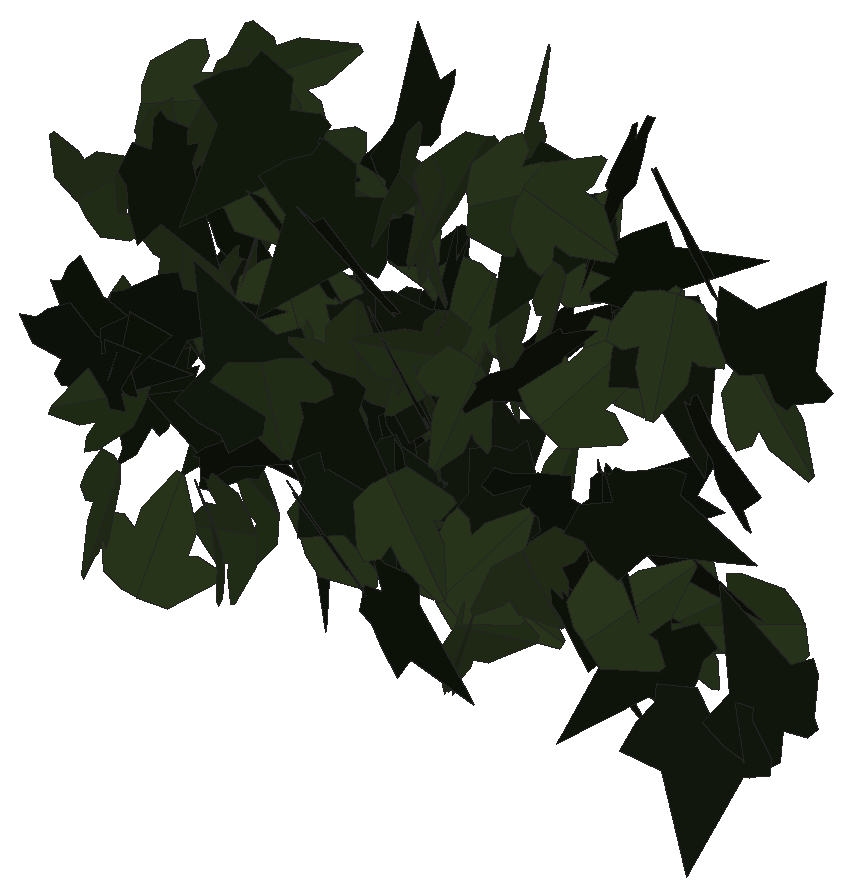
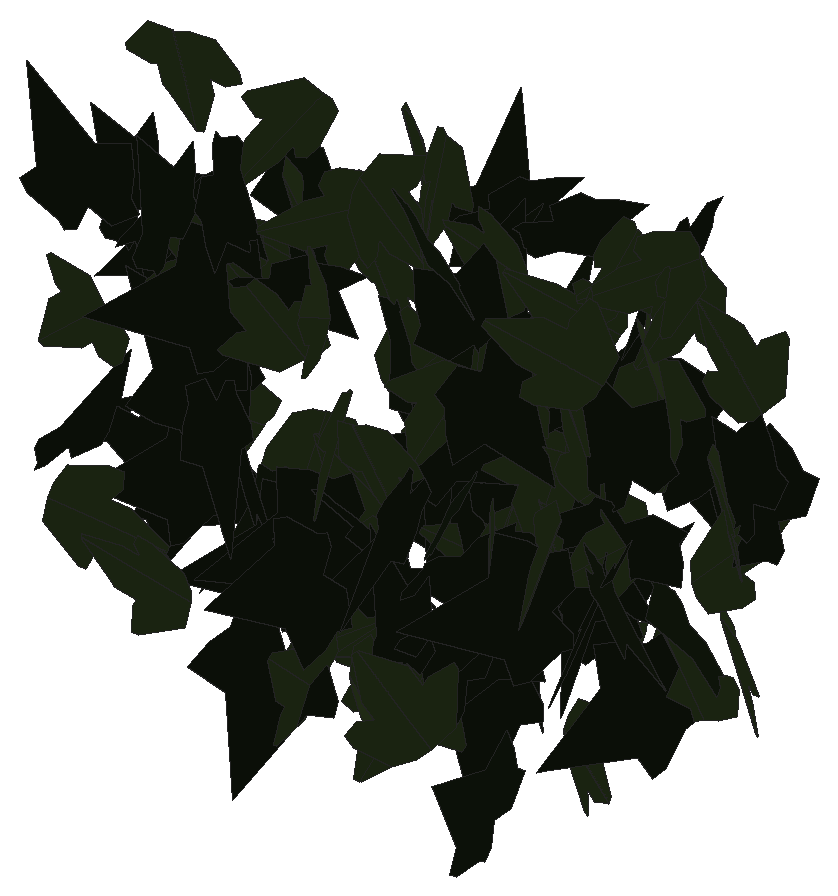
# SketchUp Ruby script. Lengths in inches.
U = 1.inch
M = Sketchup.active_model
def pt(a) = Geom::Point3d.new(a.map { |v| v * U })
def face(e, loops, mat)
  f = e.add_face(loops[0].map { |a| pt(a) })
  loops[1..].each { |l| e.add_face(l.map { |a| pt(a) }).erase! }
  f.material = f.back_material = mat if mat
  f
end
# faces: each face lists its corners as indices into pts; further lists are holes
def faces(e, pts, list, mat = nil) = list.each { |f| face(e, (f[0].is_a?(Array) ? f : [f]).map { |l| l.map { |i| pts[i] } }, mat) }
# xy, xz, yz: faces in a plane at the given z, y or x. An outline is a flat list of corners, or four numbers for a rectangle; further outlines are holes
def ring(l) = l.size == 4 ? [[l[0], l[1]], [l[2], l[1]], [l[2], l[3]], [l[0], l[3]]] : l.each_slice(2).to_a
def flat(e, list, mat, &to3) = list.each { |f| face(e, (f[0].is_a?(Array) ? f : [f]).map { |l| ring(l).map { |u, v| to3.(u, v) } }, mat) }
def xy(e, z, list, mat = nil) = flat(e, list, mat) { |x, y| [x, y, z] }
def xz(e, y, list, mat = nil) = flat(e, list, mat) { |x, z| [x, y, z] }
def yz(e, x, list, mat = nil) = flat(e, list, mat) { |y, z| [x, y, z] }
def lines(e, pts, list) = list.each { |a, b| e.add_line(pt(pts[a]), pt(pts[b])) }
# prism: a flat outline (further loops are holes) pulled along v
def prism(e, loops, v, mat = nil)
  f = face(e, loops, mat); d = Geom::Vector3d.new(v.map { |x| x * U })
  f.pushpull(f.normal.samedirection?(d) ? d.length : -d.length)
end
def box(e, o, s, mat = nil) = prism(e, [[o, [o[0] + s[0], o[1], o[2]], [o[0] + s[0], o[1] + s[1], o[2]], [o[0], o[1] + s[1], o[2]]]], [0, 0, s[2]], mat)
def at(x, y, z, deg = 0) = Geom::Transformation.translation(pt([x, y, z])) * Geom::Transformation.rotation(ORIGIN, Z_AXIS, deg.degrees)
def axes(o, x, y, z) = Geom::Transformation.new([*x, 0, *y, 0, *z, 0, *pt(o).to_a, 1])
def part(name) = M.definitions.add(name)
# library, detail: a bought-in or finely detailed component or shape, given as its bounding box
def library(name, o, s) = part(name).tap { |d| box(d.entities, o, s) }
def detail(e, o, s) = box(e.add_group.entities, o, s)
def put(e, d, t, mat = nil) = e.add_instance(d, t).tap { |i| i.material = mat if mat }
def group(e, t, mat = nil) = e.add_group.tap { |g| g.transformation = t; g.material = mat if mat }.entities
root = M.entities
M.materials.add("efeu1").color = [18, 25, 13]
M.materials.add("efeu2").color = [43, 57, 29]
c1 = part("ivyleaf_9")
p = [[1.54,2.16,1.25],[1.36,2.04,1.19],[-0.21,0.99,0.68],[-0.71,1.11,0.82],[-0.85,0.86,0.67],[-0.8,0.17,0.21],
  [-0.9,-0.01,0.1],[-0.67,-0.16,-0.02],[-0.08,-0.08,-0.05],[-0.03,-0.6,-0.4],[0.65,-0.88,-0.66],[0.83,-0.6,-0.49],
  [1.29,-0.42,-0.43],[1.8125,-0.07,-0.26],[1.21,0.44,0.15]]
faces(c1.entities,p,[[0,1,2,3,4,5,6,7,8,9,10,11,12,13,14]],"efeu1")
c2 = part("ivyleaf_10")
p = [[0,0.5,-0.03],[-0.0625,2.02,-0.43],[-0.19,2.01,-0.46],[-0.54,1.05,-0.29],[-0.52,0.625,-0.18],[-0.83,0.76,-0.28],
  [-1.16,0.64,-0.33],[-1.15,0.33,-0.24],[-0.77,-0.39,0.02],[-0.3,-0.51,0.16],[0.04,-0.48,0.23],[-0.02,2.01,-0.4375],
  [-0.06,2.01,-0.43],[0.04,-0.49,0.23],[0.67,-0.49,0.14],[1.38,0.36,-0.2],[1.375,0.51,-0.24],[0.81,0.65,-0.19],
  [0.62,0.59,-0.15],[0.6,1.09,-0.28],[0.5,1.23,-0.31]]
faces(c2.entities,p,[[0,1,2,3,4,5,6,7,8,9,10],[11,12,0,13,14,15,16,17,18,19,20]],"efeu2")
put(root,c1,axes([34.07,223.39,206.13],[0.4384,-0.24034,-0.00644],[0.00838,0.00189,0.49993],[-0.24028,-0.43844,0.00568]))
put(root,c1,axes([31.94,223.07,206.74],[0.22056,-0.30024,-0.33348],[-0.20029,0.26664,-0.37254],[0.40154,0.29792,-0.00265]))
put(root,c1,axes([30.77,223.2,204.06],[0.1906,-0.09686,0.45198],[0.42903,-0.14491,-0.21197],[0.17206,0.46863,0.02787]))
put(root,c1,axes([34.6,223.26,202.79],[0.0717,-0.0025,-0.49483],[0.47484,0.14103,0.06809],[0.13923,-0.47969,0.02259]))
put(root,c2,axes([33.21,223.19,204.7],[-0.40616,-0.28493,-0.06203],[0.05046,0.03608,-0.49614],[0.2872,-0.40929,-0.00056]))
put(root,c1,axes([30.91,223.38,204.3],[0.05748,-0.04069,0.49501],[0.3527,-0.34752,-0.06953],[0.34971,0.35718,-0.01125]))
put(root,c1,axes([33.08,223.3,204.41],[-0.29967,-0.38714,0.10159],[0.07084,0.07361,0.48945],[-0.39393,0.30774,0.01073]))
put(root,c1,axes([37.58,223.06,204.92],[0.02345,0.04725,-0.49721],[0.20159,0.45452,0.0527],[0.45696,-0.20293,0.00226]))
put(root,c2,axes([35.47,223.38,205.33],[0.45672,-0.16892,-0.11347],[-0.1029,0.04882,-0.48686],[0.17556,0.46806,0.00983]))
put(root,c2,axes([31.09,223.42,202.68],[0.36787,-0.33824,-0.01633],[-0.01131,0.01182,-0.49973],[0.33844,0.36804,0.00105]))
put(root,c2,axes([31.08,223.71,203.58],[-0.01321,0.12806,0.48314],[0.05546,-0.47995,0.12873],[0.49674,0.05699,-0.00152]))
put(root,c1,axes([38.33,223.51,202.61],[-0.33617,-0.30777,-0.2056],[0.15204,0.13841,-0.45577],[0.33746,-0.36895,0.00053]))
put(root,c1,axes([33.8125,223.7,206.63],[-0.29437,-0.37516,0.15034],[-0.09391,-0.11741,-0.47686],[0.3931,-0.30898,-0.00134]))
put(root,c2,axes([34.64,223.34,203.78],[0.38218,0.0878,0.3102],[0.2955,0.09696,-0.39151],[-0.12891,0.48259,0.02222]))
put(root,c2,axes([37.89,223.44,206.87],[0.49581,0.06396,-0.00897],[-0.00898,-0.00046,-0.49992],[-0.06396,0.49589,0.0007]))
put(root,c1,axes([33.59,223.33,203.33],[0.45984,-0.15266,-0.12345],[-0.11699,0.03941,-0.48452],[0.15766,0.47449,0.00053]))
put(root,c1,axes([31.59,223.2,204.81],[0.11228,0.265,-0.40886],[0.15349,0.37898,0.28778],[0.46242,-0.19013,0.00375]))
put(root,c1,axes([36.2,223.23,205.86],[0.11141,0.48401,0.05764],[0.01045,0.05674,-0.49666],[-0.48732,0.11188,0.00253]))
put(root,c2,axes([31.14,223.57,204.49],[0.30433,-0.39325,-0.05231],[-0.02972,0.04314,-0.49725],[0.3956,0.30577,0.00288]))
put(root,c2,axes([30.74,223.57,205.66],[-0.35078,-0.05237,0.35244],[0.34824,0.05427,0.35466],[-0.0754,0.49428,-0.00159]))
put(root,c2,axes([32.18,223.72,202.19],[-0.3085,0.23753,0.3137],[0.25062,-0.18868,0.38934],[0.30334,0.39746,-0.00264]))
put(root,c1,axes([38.12,223.85,205.24],[0.08623,-0.14365,0.47109],[0.23735,-0.40694,-0.16753],[0.43155,0.25252,-0.00199]))
put(root,c2,axes([31.5,223.5,201.88],[0.45195,0.15396,-0.14845],[0.13309,0.06923,0.47696],[0.16742,-0.47064,0.02159]))
put(root,c2,axes([34.88,223.61,207.05],[0.30292,-0.3586,-0.17218],[-0.10876,0.13351,-0.46941],[0.38263,0.32184,0.00289]))
put(root,c2,axes([31.86,223.68,205.34],[-0.47292,0.00245,0.1623],[-0.16231,-0.00107,-0.47292],[-0.00197,-0.49999,0.00181]))
put(root,c1,axes([33.3125,223.76,204.23],[0.0215,-0.10125,-0.48917],[0.44127,0.23334,-0.0289],[0.23413,-0.43047,0.09938]))
put(root,c1,axes([32.73,224.0625,207.03],[-0.3723,-0.31172,0.11928],[-0.09291,-0.07484,-0.48556],[0.32057,-0.38371,-0.00219]))
put(root,c2,axes([31.5,223.47,206.47],[-0.09083,-0.25316,-0.4215],[0.11357,0.40624,-0.26846],[0.47839,-0.1445,-0.01629]))
put(root,c2,axes([32.52,223.62,202.6],[0.17773,-0.10158,-0.45617],[-0.3627,0.27779,-0.20317],[0.29472,0.40313,0.02506]))
put(root,c1,axes([36.63,224.04,204.18],[0.06684,-0.04272,-0.49367],[0.49048,-0.06511,0.07204],[-0.07045,-0.4939,0.03321]))
put(root,c2,axes([31.4375,224.16,205.71],[0.00836,-0.11522,-0.48647],[0.24776,-0.42163,0.10412],[-0.43422,-0.2428,0.05004]))
put(root,c2,axes([35.12,223.84,202.42],[0.22829,-0.4181,-0.1519],[-0.05943,0.14054,-0.47615],[0.44085,0.23546,0.01447]))
put(root,c1,axes([33.84,223.89,203.62],[-0.14546,-0.31251,-0.36219],[0.18397,0.3129,-0.34387],[0.44158,-0.2333,0.02396]))
put(root,c2,axes([33.68,223.95,204.54],[-0.49079,-0.07993,0.05232],[0.05206,0.00584,0.49725],[-0.0801,0.49354,0.00259]))
put(root,c2,axes([35.92,223.78,203.39],[-0.21641,-0.40029,-0.2072],[0.10442,0.17907,-0.45501],[0.43848,-0.24021,0.00609]))
put(root,c2,axes([35.08,223.82,202.9],[0.39783,-0.05889,-0.29709],[0.30247,0.05209,0.39471],[-0.01554,-0.49378,0.07707]))
put(root,c2,axes([36.97,223.63,203.15],[0.24053,0.10153,-0.42642],[0.31555,0.29752,0.24882],[0.30426,-0.38881,0.07905]))
put(root,c2,axes([33.43,223.79,202.79],[-0.15112,-0.09875,0.46627],[0.37788,0.27328,0.18035],[-0.29047,0.4069,-0.00797]))
put(root,c2,axes([34.38,224.31,204.86],[-0.16062,-0.14724,-0.45002],[-0.25648,-0.3724,0.21339],[-0.39802,0.2994,0.0441]))
put(root,c2,axes([35.98,224.08,206.17],[0.33213,-0.37264,0.02882],[0.01921,-0.02148,-0.49917],[0.37326,0.33269,0.00005]))
put(root,c2,axes([34.26,224.2,206.37],[0.11398,-0.16037,0.45966],[0.43291,-0.18257,-0.17104],[0.2227,0.43698,0.09724]))
put(root,c1,axes([37.16,224.32,202.8],[-0.04519,0.04954,-0.49548],[0.10819,-0.48466,-0.05832],[-0.48606,-0.11248,0.03308]))
put(root,c2,axes([34.39,224.1875,204.21],[-0.26461,0.1229,0.40605],[0.35228,-0.203,0.29102],[0.23639,0.4401,0.02084]))
put(root,c2,axes([36.3,223.77,205.24],[0.30242,0.13345,-0.37514],[0.29554,0.24045,0.32379],[0.26683,-0.41758,0.06656]))
put(root,c2,axes([34.34,223.8,207.04],[0.03312,-0.33798,-0.36697],[-0.039,0.3649,-0.3396],[0.49737,0.05112,-0.00219]))
put(root,c1,axes([34.13,223.88,205.06],[0.39342,-0.07811,-0.29853],[-0.28881,0.07717,-0.40079],[0.10868,0.4878,0.0156]))
put(root,c1,axes([32.45,223.71,203.56],[0.25626,0.39871,0.15927],[0.08787,0.13285,-0.47395],[-0.42025,0.27089,-0.00198]))
put(root,c1,axes([38.73,224.08,202.48],[-0.21119,-0.41637,0.17899],[0.07731,0.16148,0.46685],[-0.44657,0.22486,-0.00383]))
put(root,c1,axes([32.7,224.39,205.41],[0.35135,-0.35568,0.00652],[-0.00459,0.00464,0.49996],[-0.35571,-0.35138,-0.00001]))
put(root,c2,axes([31.46,223.83,206.85],[-0.02544,-0.08901,-0.49136],[0.34034,0.35693,-0.08228],[0.36541,-0.33864,0.04243]))
put(root,c2,axes([35.15,223.84,202.41],[-0.09021,-0.25578,-0.42005],[0.15535,0.39037,-0.27107],[0.46661,-0.17942,0.00904]))
put(root,c1,axes([33.62,224.3,203.6],[-0.14995,-0.0359,-0.47563],[0.47558,0.02703,-0.15197],[0.03662,-0.49798,0.02604]))
put(root,c1,axes([36.16,224.09,202.86],[0.41553,-0.24357,-0.13418],[-0.11019,0.07731,-0.48154],[0.25533,0.42976,0.01057]))
put(root,c2,axes([33.18,224.29,206.43],[0.00177,0.00283,-0.49999],[0.44477,-0.22842,0.00028],[-0.22842,-0.44476,-0.00333]))
put(root,c2,axes([32.27,224.06,206.05],[0.25037,-0.02872,-0.43185],[0.42726,0.09595,0.24133],[0.06901,-0.48987,0.07259]))
put(root,c2,axes([31.94,223.97,206.92],[-0.03508,-0.28814,-0.40712],[0.0865,0.39843,-0.28944],[0.49121,-0.09074,0.02189]))
put(root,c1,axes([31.99,224.59,203.04],[0.01665,0.00497,0.4997],[-0.392,-0.30996,0.01614],[0.30994,-0.3923,-0.00642]))
put(root,c1,axes([33.5625,224.66,203.77],[0.04799,-0.34459,0.35911],[0.03588,-0.35744,-0.34778],[0.4964,0.05915,-0.00958]))
put(root,c2,axes([35.88,224.0625,207.15],[0.08648,0.33064,0.36497],[0.08023,0.35614,-0.34165],[-0.48589,0.11765,0.00854]))
put(root,c1,axes([33.42,224.49,205.6875],[0.39266,-0.06735,0.30213],[-0.29523,0.06521,0.39823],[-0.09305,-0.49113,0.01144]))
put(root,c1,axes([31.14,224.0625,203.125],[-0.3581,0.30239,-0.17414],[-0.1335,0.11182,0.46869],[0.3224,0.38217,0.00065]))
put(root,c2,axes([34.52,224.65,206.93],[0.01234,-0.43248,0.25062],[0.0019,-0.25065,-0.43263],[0.49984,0.01163,-0.00454]))
put(root,c1,axes([36.65,224.41,203.99],[0.38756,0.31035,-0.05901],[0.04133,0.04279,0.49645],[0.31319,-0.38969,0.00751]))
put(root,c1,axes([37,224.56,205.99],[0.04974,-0.46674,-0.17226],[-0.01821,0.1713,-0.46939],[0.49719,0.05297,0.00004]))
put(root,c1,axes([33.9375,224.76,204.55],[-0.09456,-0.11124,-0.47821],[-0.28459,-0.38442,0.14569],[-0.40008,0.29974,0.00939]))
put(root,c1,axes([32.01,224.84,203.81],[-0.41113,-0.28083,0.0459],[-0.03495,-0.03021,-0.49786],[0.2824,-0.41258,0.0052]))
put(root,c1,axes([32.62,224.73,202.73],[-0.19506,0.02643,-0.45962],[0.45732,-0.04633,-0.19675],[-0.05299,-0.49715,-0.0061]))
put(root,c1,axes([32.42,224.91,202.76],[0.11449,-0.34193,0.34638],[0.15474,-0.3118,-0.35894],[0.46146,0.18939,0.03442]))
put(root,c2,axes([36.6,224.43,205.35],[0.3567,0.23554,-0.25939],[0.21808,0.14046,0.42745],[0.27423,-0.41808,-0.00253]))
put(root,c1,axes([35.02,224.7,203.29],[-0.47854,0.12026,0.08084],[-0.07874,0.01838,-0.49342],[-0.12165,-0.48497,0.00135]))
put(root,c1,axes([31.28,224.78,205.07],[-0.10126,-0.05501,0.48654],[0.3841,-0.31706,0.04409],[0.30367,0.38268,0.10647]))
put(root,c2,axes([32.28,224.73,204.15],[0.43906,-0.23754,-0.02831],[-0.02478,0.01369,-0.4992],[0.23794,0.43976,0.00025]))
put(root,c2,axes([32.69,224.91,205.64],[-0.09555,-0.02774,-0.49],[-0.422,-0.25023,0.09646],[-0.25058,0.43199,0.0244]))
put(root,c1,axes([36.33,224.52,203.48],[-0.09554,0.02319,-0.49024],[-0.48756,0.05265,0.09751],[0.05615,0.49668,0.01255]))
put(root,c2,axes([31.88,224.69,204.95],[0.20578,-0.44901,0.07776],[-0.03267,0.07056,0.49392],[-0.45452,-0.20835,-0.0003]))
put(root,c2,axes([32.23,224.6875,204.74],[0.35938,0.31794,0.14056],[0.10071,0.09828,-0.47979],[-0.33272,0.37317,0.0066]))
put(root,c1,axes([37.97,224.82,205.76],[-0.22435,0.00566,0.44681],[0.37476,-0.2699,0.19159],[0.24335,0.42086,0.11686]))
put(root,c1,axes([35.33,224.6,202.63],[0.38188,0.03497,0.32085],[0.3205,0.0175,-0.38337],[-0.03804,0.49847,-0.00905]))
put(root,c2,axes([33.02,224.62,203.78],[-0.16222,0.45108,0.14216],[-0.054,0.13164,-0.47933],[-0.46986,-0.17087,0.00601]))
put(root,c1,axes([34.27,224.43,205.09],[-0.00781,0.19555,0.46011],[-0.04538,0.45799,-0.19542],[-0.49787,-0.04481,0.01059]))
put(root,c1,axes([31.375,224.77,204.43],[-0.13857,-0.2522,-0.40889],[0.18723,0.36356,-0.2877],[0.44243,-0.23284,-0.00632]))
put(root,c2,axes([34.84,224.5625,206.64],[0.00912,-0.02692,-0.49919],[0.32058,0.38342,-0.01482],[0.38359,-0.31979,0.02425]))
put(root,c2,axes([34.49,224.74,202.27],[0.19487,0.15919,0.43207],[0.34859,0.25553,-0.25137],[-0.30085,0.3992,-0.01139]))
put(root,c1,axes([36.37,224.95,203.34],[0.40085,-0.15359,0.25638],[0.23896,-0.09288,-0.42927],[0.17949,0.46667,-0.00106]))
put(root,c2,axes([31.42,224.62,204.18],[0.05875,-0.0265,0.49583],[-0.07987,0.49228,0.03577],[-0.49007,-0.08341,0.05361]))
put(root,c2,axes([31.96,225.04,206.25],[0.39486,-0.26454,-0.15527],[-0.1191,0.10101,-0.47499],[0.28267,0.41209,0.01675]))
put(root,c1,axes([31.68,224.93,203.9375],[0.34999,-0.03686,-0.35518],[-0.35428,0.02637,-0.35184],[0.04467,0.49794,-0.00766]))
put(root,c1,axes([33.75,224.8,206.78],[-0.37999,0.1841,-0.2678],[-0.24654,0.10512,0.4221],[0.21172,0.45283,0.01089]))
put(root,c1,axes([34.79,224.88,203.17],[0.40532,0.08675,0.27962],[0.27313,0.05992,-0.4145],[-0.10543,0.48876,0.00118]))
put(root,c1,axes([30.77,224.95,202.83],[0.48374,0.03106,0.1226],[0.12239,0.00722,-0.48474],[-0.03188,0.49898,-0.00062]))
put(root,c2,axes([33.51,225.03,202.33],[0.06392,0.02979,0.495],[0.43453,0.23712,-0.07038],[-0.23895,0.43919,0.00442]))
put(root,c1,axes([31.29,225.06,204.03],[0.28125,-0.2618,-0.31993],[-0.23626,0.21574,-0.38424],[0.33923,0.36731,-0.00235]))
put(root,c1,axes([32.63,225.34,205.91],[-0.12453,0.30599,-0.37532],[0.14118,-0.34775,-0.33036],[-0.46321,-0.18826,0.00022]))
put(root,c2,axes([31.73,225.01,202.03],[0.06425,-0.02227,-0.49535],[-0.34018,0.36143,-0.06037],[0.36076,0.34478,0.03129]))
put(root,c2,axes([37.72,225.3,202.68],[0.14309,0.00658,-0.47904],[-0.47907,0.00659,-0.143],[0.00443,0.49991,0.00819]))
put(root,c1,axes([35.03,225.58,206.24],[-0.37434,-0.32981,0.03305],[-0.02345,-0.02338,-0.4989],[0.33063,-0.37507,0.00204]))
put(root,c2,axes([34.62,225.09,204.66],[-0.23098,0.38258,0.22423],[-0.12977,0.18344,-0.44666],[-0.42404,-0.26454,0.01455]))
put(root,c1,axes([36.3,225.625,206.35],[0.07425,-0.19821,0.45299],[0.20342,-0.40526,-0.21067],[0.45067,0.21558,0.02046]))
put(root,c1,axes([35.77,225.55,207.09],[-0.21281,0.17516,-0.41717],[0.32708,-0.25899,-0.27558],[-0.31263,-0.39019,-0.00435]))
put(root,c1,axes([32.66,225.24,202.57],[0.3581,0.19668,-0.28824],[-0.25624,-0.13213,-0.40851],[-0.23686,0.44029,0.00617]))
put(root,c1,axes([31.09,225.5,204.25],[-0.39926,0.17521,-0.24474],[0.21868,-0.11049,-0.43586],[-0.20681,-0.45508,0.0116]))
put(root,c2,axes([32.99,225.26,205.64],[0.22276,0.38519,0.22806],[0.10564,0.2023,-0.44487],[-0.43499,0.24638,0.00874]))
put(root,c2,axes([36.47,225.45,202.24],[0.11999,-0.06868,-0.4805],[0.47682,-0.0759,0.12992],[-0.09079,-0.48941,0.04728]))
put(root,c2,axes([37.32,225.48,205.05],[0.31093,0.03131,0.39031],[0.38718,0.04981,-0.31243],[-0.05845,0.49653,0.00673]))
put(root,c1,axes([34.09,225.45,202.95],[-0.36015,-0.29964,0.17467],[0.13388,0.11219,0.4685],[-0.31995,0.38423,-0.00058]))
put(root,c2,axes([31.45,225.35,206.39],[-0.17827,-0.16865,0.43563],[0.32435,0.29087,0.24534],[-0.33618,0.37007,0.00569]))
put(root,c2,axes([33.88,225.56,204.8],[0.46062,-0.10886,-0.16118],[-0.1553,0.04362,-0.47327],[0.1171,0.48605,0.00637]))
put(root,c1,axes([32.57,225.74,204.11],[-0.08886,-0.48699,-0.07031],[0.01968,0.06788,-0.49498],[0.49165,-0.09074,0.00711]))
put(root,c2,axes([34.93,225.47,205.54],[0.39722,0.09566,-0.28821],[0.28099,0.06415,0.40857],[0.11514,-0.48655,-0.0028]))
put(root,c1,axes([35.68,225.42,205.71],[0.27782,0.11073,0.40069],[0.3581,0.18103,-0.29832],[-0.21114,0.45273,0.02128]))
put(root,c1,axes([32.36,225.98,202.96],[0.15904,-0.22227,0.41869],[0.25358,-0.33324,-0.27322],[0.40051,0.29925,0.00673]))
put(root,c1,axes([32.98,226.13,203.05],[-0.03893,-0.05137,0.49583],[0.24257,-0.43643,-0.02616],[0.43548,0.23851,0.0589]))
put(root,c2,axes([32.26,225.64,204.39],[0.08581,-0.21931,-0.44106],[-0.16091,0.41067,-0.2355],[0.46556,0.18236,-0.0001]))
put(root,c1,axes([32.25,226.01,203.43],[-0.17672,-0.33925,-0.32199],[0.16732,0.27557,-0.38218],[0.43678,-0.24283,0.01613]))
put(root,c1,axes([33.18,225.84,204.5625],[0.15182,-0.05383,-0.47334],[-0.33164,0.34471,-0.14557],[0.342,0.35816,0.06896]))
put(root,c1,axes([34.61,225.98,202.4],[0.30454,0.39263,-0.05566],[-0.04085,-0.03874,-0.49682],[-0.39445,0.30715,0.00848]))
put(root,c2,axes([32.89,226.13,202.65],[-0.38308,-0.22994,-0.22444],[0.19868,0.10498,-0.44666],[0.25253,-0.4314,0.01094]))
put(root,c2,axes([31.37,225.93,204.78],[-0.11958,0.1535,0.46058],[-0.26927,0.37373,-0.19447],[-0.40397,-0.29456,-0.00671]))
put(root,c2,axes([34.08,226.08,206.36],[0.1616,-0.21161,0.42321],[-0.27553,0.32149,0.26595],[-0.38467,-0.31917,-0.0127]))
put(root,c2,axes([34.25,226,202.24],[0.02187,0.31057,-0.39124],[0.04917,0.38838,0.31104],[0.4971,-0.05208,-0.01355]))
put(root,c1,axes([35.22,226.23,205.04],[0.24784,0.03647,-0.43272],[-0.42945,-0.05333,-0.25046],[-0.06442,0.49581,0.00489]))
put(root,c1,axes([31.1,226.3,204.27],[0.37776,0.03737,0.32543],[0.32026,0.06216,-0.3789],[-0.06878,0.49471,0.02303]))
put(root,c2,axes([32.84,226.97,203.09],[0.26632,-0.32374,0.27252],[0.1694,-0.21351,-0.41919],[0.38778,0.31561,-0.00404]))
put(root,c1,axes([33.85,226.38,203.72],[-0.07568,0.32938,-0.36848],[-0.10929,0.35239,0.33745],[0.482,0.13162,0.01866]))
put(root,c1,axes([31.15,227.08,202.3],[0.23515,-0.31311,0.31091],[0.18118,-0.25272,-0.39154],[0.40234,0.29681,-0.0054]))
put(root,c2,axes([32.15,227.02,202.92],[-0.19067,-0.396,0.23839],[0.10031,0.21628,0.4395],[-0.4512,0.21542,-0.00303]))
